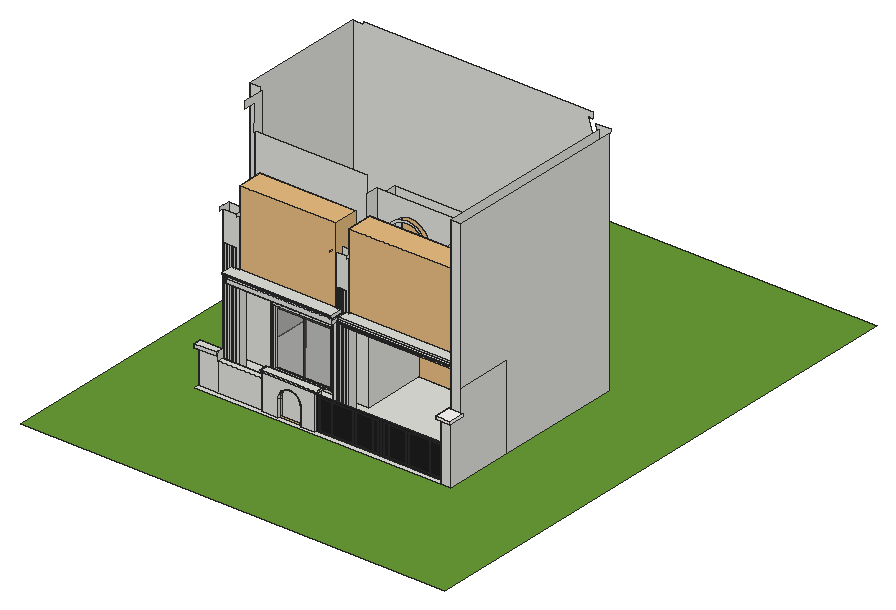
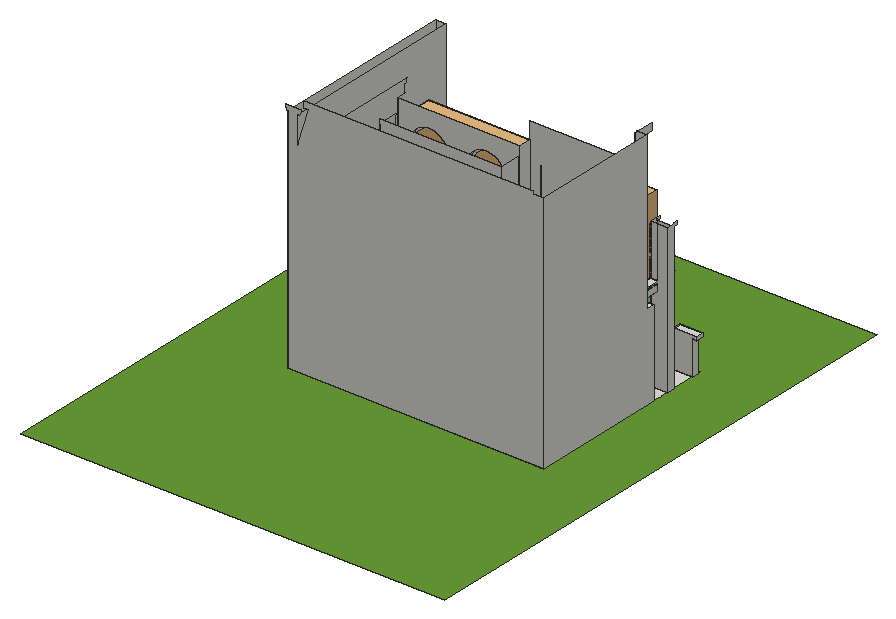
# SketchUp Ruby script. Lengths in millimetres.
U = 1.mm
M = Sketchup.active_model
def pt(a) = Geom::Point3d.new(a.map { |v| v * U })
def face(e, loops, mat)
  f = e.add_face(loops[0].map { |a| pt(a) })
  loops[1..].each { |l| e.add_face(l.map { |a| pt(a) }).erase! }
  f.material = f.back_material = mat if mat
  f
end
# faces: each face lists its corners as indices into pts; further lists are holes
def faces(e, pts, list, mat = nil) = list.each { |f| face(e, (f[0].is_a?(Array) ? f : [f]).map { |l| l.map { |i| pts[i] } }, mat) }
# xy, xz, yz: faces in a plane at the given z, y or x. An outline is a flat list of corners, or four numbers for a rectangle; further outlines are holes
def ring(l) = l.size == 4 ? [[l[0], l[1]], [l[2], l[1]], [l[2], l[3]], [l[0], l[3]]] : l.each_slice(2).to_a
def flat(e, list, mat, &to3) = list.each { |f| face(e, (f[0].is_a?(Array) ? f : [f]).map { |l| ring(l).map { |u, v| to3.(u, v) } }, mat) }
def xy(e, z, list, mat = nil) = flat(e, list, mat) { |x, y| [x, y, z] }
def xz(e, y, list, mat = nil) = flat(e, list, mat) { |x, z| [x, y, z] }
def yz(e, x, list, mat = nil) = flat(e, list, mat) { |y, z| [x, y, z] }
def lines(e, pts, list) = list.each { |a, b| e.add_line(pt(pts[a]), pt(pts[b])) }
# prism: a flat outline (further loops are holes) pulled along v
def prism(e, loops, v, mat = nil)
  f = face(e, loops, mat); d = Geom::Vector3d.new(v.map { |x| x * U })
  f.pushpull(f.normal.samedirection?(d) ? d.length : -d.length)
end
def box(e, o, s, mat = nil) = prism(e, [[o, [o[0] + s[0], o[1], o[2]], [o[0] + s[0], o[1] + s[1], o[2]], [o[0], o[1] + s[1], o[2]]]], [0, 0, s[2]], mat)
def at(x, y, z, deg = 0) = Geom::Transformation.translation(pt([x, y, z])) * Geom::Transformation.rotation(ORIGIN, Z_AXIS, deg.degrees)
def axes(o, x, y, z) = Geom::Transformation.new([*x, 0, *y, 0, *z, 0, *pt(o).to_a, 1])
def part(name) = M.definitions.add(name)
# library, detail: a bought-in or finely detailed component or shape, given as its bounding box
def library(name, o, s) = part(name).tap { |d| box(d.entities, o, s) }
def detail(e, o, s) = box(e.add_group.entities, o, s)
def put(e, d, t, mat = nil) = e.add_instance(d, t).tap { |i| i.material = mat if mat }
def group(e, t, mat = nil) = e.add_group.tap { |g| g.transformation = t; g.material = mat if mat }.entities
root = M.entities
M.materials.add("[0010_Snow]").color = [255, 250, 250]
M.materials.add("[Asphalt New]").color = [67, 60, 62]
M.materials.add("[Color M08]").color = [30, 30, 30]
M.materials.add("[Grass Dark Green]").color = [106, 157, 55]
M.materials.add("[Translucent Glass Gray]").color = [128, 128, 128]
M.materials["[Translucent Glass Gray]"].alpha = 0.5
M.materials.add("[Wood Floor]").color = [155, 105, 61]
M.materials.add("[Wood OSB]").color = [240, 195, 122]
c1 = part("Group\#102")
g1 = group(c1.entities,at(0,0,0))
prism(g1,[[[0,76.2,1828.8],[1790.7,76.2,1828.8],[1790.7,76.2,0],[0,76.2,0]],[[1714.5,76.2,76.2],[1714.5,76.2,1752.6],[76.2,76.2,1752.6],[76.2,76.2,76.2]]],[0,-76.2,0])
c2 = part("Group\#135")
box(c2.entities,[0,0,0],[12.7,25.4,1676.4])
c3 = part("Double driveway gate")
g2 = group(c3.entities,at(1790.7,0,0),"[Color M08]")
put(g2,c1,axes([1790.7,0,0],[-1,0,0],[0,1,0],[0,0,1]))
g3 = group(g2,at(76.2,50.8,76.2))
g4 = group(g3,at(0,-25.4,0))
box(g4,[0,0,0],[139.8,25.4,1676.4])
box(g4,[1291.2,0,0],[347.1,25.4,1676.4])
box(g4,[712.6,0,0],[565.9,25.4,1676.4])
box(g4,[626.3,0,0],[73.6,25.4,1676.4])
box(g4,[152.5,0,0],[461.1,25.4,1676.4])
put(g3,c2,axes([1278.5,0,0],[1,0,0],[0,-1,0],[0,0,1]))
put(g3,c2,axes([613.6,0,0],[1,0,0],[0,-1,0],[0,0,1]))
put(g3,c2,axes([699.9,0,0],[1,0,0],[0,-1,0],[0,0,1]))
put(g3,c2,axes([139.8,0,0],[1,0,0],[0,-1,0],[0,0,1]))
g5 = group(c3.entities,at(1790.7,0,0),"[Color M08]")
put(g5,c1,at(-1790.7,0,0))
g6 = group(g5,at(-76.2,50.8,76.2,-180))
g7 = group(g6,at(0,25.4,0))
box(g7,[0,-25.4,0],[139.8,25.4,1676.4])
box(g7,[1291.2,-25.4,0],[347.1,25.4,1676.4])
box(g7,[712.6,-25.4,0],[565.9,25.4,1676.4])
box(g7,[626.3,-25.4,0],[73.6,25.4,1676.4])
box(g7,[152.5,-25.4,0],[461.1,25.4,1676.4])
put(g6,c2,at(1278.5,0,0))
put(g6,c2,at(613.6,0,0))
put(g6,c2,at(699.9,0,0))
put(g6,c2,at(139.8,0,0))
c4 = library("Glazed entrance door",[0,-35,0],[1000,80.2,2000])
c5 = library("escalier+0",[0,-20,30],[1600,1520,2232])
xy(root,0,[[18830,7763.7,19424.7,7763.7,19424.7,19554.1,4179.9,19554.1,4179.9,11364.2,11672.4,11364.2,11672.4,15798,13910.6,15798,13910.6,15291.6,14018.3,15291.6,14018.3,15102.7,18830,15102.7],[4179.9,7763.7,18830,7763.7,18830,8093.7,11165.5,8093.7,11165.5,7988.9,10315.5,7988.9,10315.5,8071.5,8985.2,8071.5,8985.2,7988.9,8014.2,7988.9,8014.2,8093.7,4179.9,8093.7],[11165.5,8093.7,18830,8932],[[4179.9,8420.8,11165.5,8420.8,11165.5,8932,18830,8932,18830,15102.7,13910.6,15102.7,13910.6,15291.6,11672.4,15291.6,11672.4,11364.2,9781,11364.2,9781,11351.5,9666.6,11351.5,9666.6,11288,5975.6,11288,5975.6,11351.5,5861.2,11351.5,5861.2,11364.2,4179.9,11364.2,4179.9,10323.8,5191.1,10323.8,5191.1,9852.4,4980.7,9852.4,4980.7,10104.8,4850.6,10104.8,4850.6,9852.4,4702.2,9852.4,4702.2,10104.8,4585.1,10104.8,4585.1,9852.4,4415.9,9852.4,4415.9,10085.7,4330.2,10085.7,4330.2,9852.4,4179.9,9852.4],[10715.6,9852.4,10715.6,10323.8,11726.9,10323.8,11726.9,9852.4,11548,9852.4,11548,9993.6,11425.8,9993.6,11425.8,9852.4,11289.9,9852.4,11289.9,10007.9,11185.3,10007.9,11185.3,9852.4,11053.6,9852.4,11053.6,10033.3,10956.8,10033.3,10956.8,9852.4]],[4179.9,9852.4,4330.2,9852.4,4330.2,10085.7,4415.9,10085.7,4415.9,9852.4,4585.1,9852.4,4585.1,10104.8,4702.2,10104.8,4702.2,9852.4,4850.6,9852.4,4850.6,10104.8,4980.7,10104.8,4980.7,9852.4,5191.1,9852.4,5191.1,10323.8,4179.9,10323.8],
  [5975.6,11288,9666.6,11364.2],[5861.2,11351.5,5975.6,11364.2],[9666.6,11351.5,9781,11364.2],[13910.6,15102.7,14018.3,15291.6],[11672.4,15291.6,13910.6,15798]])
xy(root,0,[[[0,0,25274.6,32180.2],[4179.9,7763.7,4179.9,8093.7,8014.2,8093.7,8014.2,7988.9,8985.2,7988.9,8985.2,8071.5,10315.5,8071.5,10315.5,7988.9,11165.5,7988.9,11165.5,8420.8,4179.9,8420.8,4179.9,19554.1,19424.7,19554.1,19424.7,7763.7]]],"[Grass Dark Green]")
xy(root,66,[[9051.2,8071.5,10249.5,8133.4]],"[Wood OSB]")
xy(root,122.4,[[6098,11288,9544.2,11335.6]])
xy(root,199.8,[[6175.4,11335.6,9466.7,11364.2]])
xy(root,359.4,[[15054.6,15102.7,17168.6,15225]])
xy(root,478.1,[[15173.4,15225,17049.8,15291.6]])
xy(root,1708.2,[[5311.7,8093.7,8014.2,8420.8]])
xy(root,2001,[[3987.8,7966.7,5311.7,8093.7],[3987.8,8093.7,4179.9,8420.8]])
xy(root,2102.1,[[7968.2,7949.2,7968.2,8093.7,8014.2,8093.7,8014.2,7988.9,11165.5,7988.9,11165.5,8093.7,11262.4,8093.7,11262.4,7949.2],[7968.2,8093.7,8014.2,8420.8],[11165.5,8093.7,11262.4,8420.8]])
xy(root,2185.3,[[7917.4,7919.1,11392.6,7949.2],[7917.4,7949.2,7968.2,8420.8],[11262.4,7949.2,11392.6,8420.8]])
xy(root,2213,[[7917.4,7919.1,11392.6,8420.8],[3987.8,7966.7,5311.7,8420.8]])
xy(root,3491.1,[[6175.4,11335.6,9466.7,11364.2]])
xy(root,3501.3,[[18683.9,7590.7,18830,8551.1],[18830,7590.7,19424.7,7763.7],[19424.7,7590.7,19532.6,8551.1]])
xy(root,3568.6,[[6098,11288,9544.2,11335.6]])
xy(root,3679.7,[[18683.9,7590.7,19532.6,8551.1]],"[0010_Snow]")
xy(root,3690.9,[[5975.6,11288,9666.6,11351.5]])
xy(root,3756.3,[[15173.4,15225,17049.8,15291.6]])
xy(root,3765.6,[[11672.4,15102.7,11780.1,15291.6],[11780.1,15102.7,13910.6,15798],[11672.4,15291.6,11780.1,15798]])
xy(root,3805.4,[[5861.2,11351.5,9781,11364.2]])
xy(root,3873.3,[[11672.4,15102.7,11780.1,15291.6]])
xy(root,3875.1,[[15054.6,15102.7,17168.6,15225]])
xy(root,4860.9,[[11672.4,9994.1,18830,15102.7]],"[Wood Floor]")
xy(root,4981.6,[[11545.3,9700.5,11545.3,11364.2,11672.4,11364.2,11672.4,9994.1,18830,9994.1,18830,9700.5]])
xy(root,5014.6,[[5191.1,11364.2,10815.6,11889.6]])
xy(root,5014.6,[[5191.1,9487.7,10815.6,11364.2]],"[Wood Floor]")
xy(root,5151.1,[[4815.5,9262.3,4815.5,11364.2,5191.1,11364.2,5191.1,9487.7,10815.6,9487.7,10815.6,11364.2,11160.4,11364.2,11160.4,9262.3],[4179.9,11364.2,4815.5,11889.6],[4815.5,11364.2,5191.1,11889.6],[10815.6,11364.2,11160.4,11889.6]])
xy(root,5371.1,[[11545.3,9262.3,18830,9700.5]])
xy(root,5459.8,[[4802.8,9262.3,4815.5,9852.4],[11160.4,9262.3,11216,9852.4]])
xy(root,5528.1,[[11545.3,9136.9,18830,9262.3]])
xy(root,5565.8,[[11545.3,9136.9,18830,9495.7]])
xy(root,5593.4,[[4747.3,9214.7,11271.6,9262.3],[4747.3,9262.3,4802.8,9852.4],[11216,9262.3,11271.6,9852.4],[4747.3,9852.4,4815.5,11889.6],[11160.4,9852.4,11271.6,11364.2],
  [11160.4,11364.2,11271.6,11889.6]])
xy(root,5638,[[4747.3,9152.8,11271.6,9214.7]])
xy(root,5663.2,[[11545.3,9194,18830,9495.7]])
xy(root,5726.3,[[4747.3,9062.3,11271.6,9152.8]])
xy(root,5732,[[11545.3,9194,18830,9194,18830,12124.7,18102.6,12124.7,18102.6,11848.5,15805,11848.5,15805,12124.7,14682.1,12124.7,14682.1,11848.5,12388.2,11848.5,12388.2,12124.7,11545.3,12124.7],[11545.3,12281.7,18830,12281.7,18830,13477.1,14275.5,13477.1,14275.5,14659.8,11972,14659.8,11972,13477.1,11545.3,13477.1]])
xy(root,5760.6,[[4747.3,9062.3,11271.6,9062.3,11271.6,10323.8,10715.6,10323.8,10715.6,10381,5191.1,10381,5191.1,9852.4,4747.3,9852.4],[4747.3,10323.8,5191.1,10323.8,5191.1,10381,10715.6,10381,10715.6,10323.8,11271.6,10323.8,11271.6,11364.2,9713.9,11364.2,9713.9,11161,9599.1,11161,9599.1,11195.9,9482.2,11195.9,9482.2,11161,9386.9,11161,9386.9,11364.2,6306,11364.2,6306,11161,6210.7,11161,6210.7,11195.9,6093.9,11195.9,6093.9,11161,5979,11161,5979,11364.2,4869.5,11364.2,4869.5,11889.6,4747.3,11889.6],[5979,11161,6093.9,11364.2],[6210.7,11161,6306,11364.2],[9386.9,11161,9482.2,11364.2],
  [9599.1,11161,9713.9,11364.2],[6093.9,11195.9,6210.7,11364.2],[9482.2,11195.9,9599.1,11364.2],[4869.5,11364.2,11271.6,11889.6]])
xy(root,5839.2,[[12495.4,11848.5,14574.9,12281.7]])
xy(root,5844,[[15917.1,11848.5,17990.5,12281.7]])
xz(root,7590.7,[[18683.9,3501.3,19532.6,3679.7]],"[0010_Snow]")
xz(root,7763.7,[[18830,0,19424.7,3501.3]])
xz(root,7919.1,[[7917.4,2185.3,11392.6,2213]])
xz(root,7949.2,[[7968.2,2102.1,11262.4,2185.3]])
xz(root,7966.7,[[3987.8,2001,5311.7,2213]])
xz(root,7988.9,[[8014.2,0,8985.2,0,8985.2,1044.4,9007.8,1216.5,9074.3,1377,9150.6,1476.4,9180,1514.7,9317.7,1620.4,9478.2,1686.9,9650.3,1709.5,9822.5,1686.9,9982.9,1620.4,10120.7,1514.7,10150.1,1476.4,10226.4,1377,10292.8,1216.5,10315.5,1044.4,10315.5,0,11165.5,0,11165.5,2102.1,8014.2,2102.1]])
xz(root,8071.5,[[[8985.2,0,10315.5,0,10315.5,1044.4,10292.8,1216.5,10226.4,1377,10150.1,1476.4,10120.7,1514.7,9982.9,1620.4,9822.5,1686.9,9650.3,1709.5,9478.2,1686.9,9317.7,1620.4,9180,1514.7,9150.6,1476.4,9074.3,1377,9007.8,1216.5,8985.2,1044.4],[9051.2,66,9051.2,1040.1,9072.2,1199.3,9132,1343.7,9202.9,1436.2,9227.1,1467.6,9351,1562.8,9495.4,1622.5,9650.3,1642.9,9805.2,1622.5,9949.6,1562.8,10073.6,1467.6,10097.7,1436.2,10168.7,1343.7,10228.5,1199.3,10249.5,1040.1,10249.5,66]]],"[Wood OSB]")
xz(root,8093.7,[[4179.9,0,5311.7,2001],[5311.7,0,8014.2,1708.2]])
xz(root,8133.4,[[9051.2,66,10249.5,66,10249.5,1040.1,10228.5,1199.3,10168.7,1343.7,10097.7,1436.2,10073.6,1467.6,9949.6,1562.8,9805.2,1622.5,9650.3,1642.9,9495.4,1622.5,9351,1562.8,9227.1,1467.6,9202.9,1436.2,9132,1343.7,9072.2,1199.3,9051.2,1040.1]])
xz(root,8420.8,[[4179.9,0,4179.9,2001,3987.8,2001,3987.8,2213,5311.7,2213,5311.7,1708.2,8014.2,1708.2,8014.2,2102.1,7968.2,2102.1,7968.2,2185.3,7917.4,2185.3,7917.4,2213,11392.6,2213,11392.6,2185.3,11262.4,2185.3,11262.4,2102.1,11165.5,2102.1,11165.5,0]])
xz(root,8551.1,[[18683.9,3501.3,18830,3679.7],[19424.7,3501.3,19532.6,3679.7],[18830,3679.7,19424.7,13753.6]])
xz(root,9062.3,[[4747.3,5726.3,11271.6,5760.6]])
xz(root,9136.9,[[11545.3,5528.1,18830,5565.8]])
xz(root,9152.8,[[4747.3,5638,11271.6,5726.3]])
xz(root,9194,[[11545.3,5663.2,18830,5732]])
xz(root,9214.7,[[4747.3,5593.4,11271.6,5638]])
xz(root,9262.3,[[4815.5,5151.1,11160.4,5459.8],[11545.3,5371.1,18830,5528.1],[4802.8,5459.8,11216,5593.4]])
xz(root,9487.7,[[5191.1,5014.6,10815.6,5151.1]])
xz(root,9495.7,[[11545.3,5565.8,18830,5663.2]])
xz(root,9700.5,[[11545.3,4981.6,18830,5088.6],[11545.3,5088.6,18830,5371.1]])
xz(root,9852.4,[[4179.9,0,4330.2,6858],[4415.9,0,4585.1,6858],[[4702.2,0,4850.6,6858],[4802.8,5459.8,4815.5,5593.4]],[4980.7,0,5191.1,5760.6],[10715.6,0,10715.6,8713.5,11726.9,8713.5,11726.9,0,11548,0,11548,6872.3,11425.8,6872.3,11425.8,0,11289.9,0,11289.9,6861.6,11185.3,6861.6,11185.3,5593.4,11160.4,5593.4,11160.4,5459.8,11185.3,5459.8,11185.3,0,11053.6,0,11053.6,6858,10956.8,6858,10956.8,0],
  [4802.8,5459.8,4815.5,5593.4],[11160.4,5459.8,11185.3,5593.4],[11185.3,5459.8,11216,5593.4],[11185.3,5593.4,11216,6861.6],[4980.7,5760.6,5191.1,5760.6,5191.1,8639.6,4179.9,8639.6,4179.9,6858,4980.7,6858]])
xz(root,9993.6,[[11425.8,0,11548,6872.3]])
xz(root,9994.1,[[11672.4,4860.9,18830,4981.6]])
xz(root,10007.9,[[11185.3,0,11289.9,6861.6]])
xz(root,10033.3,[[10956.8,0,11053.6,6858]])
xz(root,10085.7,[[4330.2,0,4415.9,6858]])
xz(root,10104.8,[[4585.1,0,4702.2,6858],[4850.6,0,4980.7,6858]])
xz(root,10323.8,[[4179.9,0,4179.9,8794.8,4747.3,8794.8,4747.3,5760.6,5191.1,5760.6,5191.1,0],[10715.6,0,11726.9,5760.6],[4747.3,5760.6,5191.1,8794.8],[10715.6,5760.6,11726.9,8794.8]])
xz(root,11161,[[5979,5760.6,6093.9,5760.6,6093.9,9007,9599.1,9007,9599.1,5760.6,9713.9,5760.6,9713.9,9121.9,5979,9121.9],[6210.7,5760.6,6306,5760.6,6306,8794.9,9386.9,8794.9,9386.9,5760.6,9482.2,5760.6,9482.2,8890.1,6210.7,8890.1]])
xz(root,11195.9,[[6093.9,5760.6,6210.7,5760.6,6210.7,8890.1,9482.2,8890.1,9482.2,5760.6,9599.1,5760.6,9599.1,9007,6093.9,9007]])
xz(root,11288,[[[5975.6,0,9666.6,3690.9],[6098,122.4,9544.2,3568.6]]])
xz(root,11335.6,[[[6098,122.4,9544.2,3568.6],[6175.4,199.8,9466.7,3491.1]]])
xz(root,11351.5,[[5861.2,0,5975.6,0,5975.6,3690.9,9666.6,3690.9,9666.6,0,9781,0,9781,3805.4,5861.2,3805.4]])
xz(root,11364.2,[[5861.2,-114.5,9781,0],[4179.9,0,5861.2,0,5861.2,3805.4,9781,3805.4,9781,0,11672.4,0,11672.4,4981.6,11545.3,4981.6,11545.3,12370.5,4869.5,12370.5,4869.5,5760.6,5979,5760.6,5979,9121.9,9713.9,9121.9,9713.9,5760.6,11271.6,5760.6,11271.6,5593.4,11160.4,5593.4,11160.4,5151.1,10815.6,5151.1,10815.6,5014.6,5191.1,5014.6,5191.1,5151.1,4179.9,5151.1],[5979,5645.7,9713.9,5760.6]])
xz(root,11364.2,[[6306,5760.6,6382.4,5760.6,6382.4,8718.5,9310.6,8718.5,9310.6,5760.6,9386.9,5760.6,9386.9,8794.9,6306,8794.9],[7846.5,5760.6,7934.9,8718.5]],"[Asphalt New]")
xz(root,11364.2,[[6175.4,199.8,9466.7,3491.1],[6382.4,5760.6,7846.5,8718.5],[7934.9,5760.6,9310.6,8718.5]],"[Translucent Glass Gray]")
xz(root,11848.5,[[[12388.2,5732,14682.1,5732,14682.1,9152.2,14670.1,9472.3,14570.4,9776.7,14390.8,10042,14163.1,10232.5,14145.1,10247.6,13852.4,10377.7,13535.2,10422.2,13217.9,10377.7,12925.2,10247.6,12907.2,10232.5,12679.5,10042,12499.9,9776.7,12400.2,9472.3,12388.2,9152.2],[12495.4,5839.2,12495.4,9150.1,12506.8,9453.2,12597.2,9729,12759.9,9969.4,12976,10150.3,12982.5,10155.7,13247.7,10273.5,13535.2,10313.9,13822.6,10273.5,14087.8,10155.7,14094.3,10150.3,14310.4,9969.4,14473.2,9729,14563.5,9453.2,14574.9,9150.1,14574.9,5839.2]],[[15805,5732,18102.6,5732,18102.6,9139.4,18092.9,9462,17994.4,9769.3,17990.5,9775.1,17814.8,10037.4,17568,10245.4,17423.3,10310.1,17273.4,10377.1,16953.8,10422.2,16634.2,10377.1,16484.3,10310.1,16339.6,10245.4,16092.8,10037.4,15917.1,9775.1,15913.2,9769.3,15814.7,9462,15805,9139.4],[15917.1,5844,15917.1,9347.6,15968.2,9601.1,16080.3,9834.2,16246.5,10032.4,16456.4,10183.4,16697.2,10277.9,16953.8,10310.1,17210.4,10277.9,17451.2,10183.4,17661.1,10032.4,17827.3,9834.2,17939.4,9601.1,17990.5,9347.6,17990.5,5844]]])
xz(root,11889.6,[[5191.1,5014.6,10815.6,5014.6,10815.6,5151.1,11160.4,5151.1,11160.4,5593.4,11271.6,5593.4,11271.6,5760.6,4747.3,5760.6,4747.3,5593.4,4815.5,5593.4,4815.5,5151.1,5191.1,5151.1],[4179.9,5151.1,4815.5,5151.1,4815.5,5593.4,4747.3,5593.4,4747.3,5760.6,4869.5,5760.6,4869.5,14284.3,4775.8,14284.3,4775.8,14452.6,4179.9,14452.6]])
xz(root,12124.7,[[11545.3,5732,12388.2,5732,12388.2,9152.2,12400.2,9472.3,12499.9,9776.7,12679.5,10042,12907.2,10232.5,12925.2,10247.6,13217.9,10377.7,13535.2,10422.2,13852.4,10377.7,14145.1,10247.6,14163.1,10232.5,14390.8,10042,14570.4,9776.7,14670.1,9472.3,14682.1,9152.2,14682.1,5732,15805,5732,15805,9139.4,15814.7,9462,15913.2,9769.3,15917.1,9775.1,16092.8,10037.4,16339.6,10245.4,16484.3,10310.1,16634.2,10377.1,16953.8,10422.2,17273.4,10377.1,17423.3,10310.1,17568,10245.4,17814.8,10037.4,17990.5,9775.1,17994.4,9769.3,18092.9,9462,18102.6,9139.4,18102.6,5732,18830,5732,18830,11371.3,11545.3,11371.3]])
xz(root,13477.1,[[11545.3,5732,11972,5732,11972,9853.1,14275.5,9853.1,14275.5,5732,18830,5732,18830,10869.6,11545.3,10869.6]])
xz(root,14659.8,[[11972,5732,14275.5,9853.1]])
xz(root,15102.7,[[[14018.3,0,18830,0,18830,4860.9,11672.4,4860.9,11672.4,3873.3,14018.3,3873.3],[15054.6,359.4,17168.6,3875.1]],[13910.6,0,14018.3,0,14018.3,3873.3,11780.1,3873.3,11780.1,3765.6,13910.6,3765.6],[11672.4,3765.6,11780.1,3873.3]])
xz(root,15225,[[[15054.6,359.4,17168.6,3875.1],[15173.4,478.1,17049.8,3756.3]]])
xz(root,15291.6,[[11672.4,-107.7,14018.3,0],[11672.4,3765.6,11780.1,3873.3]])
xz(root,15291.6,[[[15173.4,478.1,17049.8,3756.3],[15223.5,528.2,16999.8,3706.3]],[16111.6,528.2,16145.9,3706.3]],"[Asphalt New]")
xz(root,15291.6,[[15223.5,528.2,16111.6,3706.3],[16145.9,528.2,16999.8,3706.3]],"[Translucent Glass Gray]")
xz(root,15798,[[11672.4,0,13910.6,3765.6]])
xz(root,19554.1,[[4179.9,0,4179.9,14452.6,4815.5,14452.6,4815.5,14595.5,18485.5,14595.5,18485.5,14236.7,18173.1,14236.7,18830,12141.6,18830,13753.6,18742.6,13753.6,18742.6,13895.1,18683.9,13895.1,18683.9,14035.1,19558,14035.1,19558,13895.1,19486.6,13895.1,19486.6,13753.6,19424.7,13753.6,19424.7,0]])
yz(root,3987.8,[[7966.7,2001,8420.8,2213]])
yz(root,4179.9,[[8093.7,0,8420.8,2001],[9852.4,0,9852.4,8639.6,9646,8639.6,9646,8850.3,9852.4,8850.3,9852.4,8794.8,10323.8,8794.8,10323.8,0],[11364.2,0,11364.2,5151.1,11889.6,5151.1,11889.6,14452.6,19554.1,14452.6,19554.1,0]])
yz(root,4330.2,[[9852.4,0,10085.7,6858]])
yz(root,4415.9,[[9852.4,0,10085.7,6858]])
yz(root,4585.1,[[9852.4,0,10104.8,6858]])
yz(root,4702.2,[[9852.4,0,10104.8,6858]])
yz(root,4802.8,[[9262.3,5459.8,9852.4,5593.4]])
yz(root,4815.5,[[9262.3,5151.1,9262.3,5459.8,9852.4,5459.8,9852.4,5593.4,11889.6,5593.4,11889.6,5151.1]])
yz(root,4850.6,[[9852.4,0,10104.8,6858]])
yz(root,4869.5,[[11364.2,5760.6,11364.2,12370.5,11300.2,12370.5,11300.2,12768.3,11364.2,12768.3,11364.2,13883.8,10648.2,13883.8,10648.2,14284.3,11889.6,14284.3,11889.6,5760.6]])
yz(root,4980.7,[[9852.4,0,10104.8,6858]])
yz(root,5191.1,[[9852.4,0,10323.8,5014.6],[9487.7,5014.6,9852.4,5151.1],[9852.4,5014.6,10323.8,5151.1],[10323.8,5014.6,11364.2,5151.1],[11364.2,5014.6,11889.6,5151.1],
  [9852.4,5151.1,10323.8,5760.6],[9852.4,5760.6,10323.8,5760.6,10323.8,8794.8,9646,8794.8,9646,8639.6,9852.4,8639.6],[10323.8,5760.6,10381,8794.8]])
yz(root,5311.7,[[8093.7,1708.2,8420.8,2213],[7966.7,2001,8093.7,2213]])
yz(root,5861.2,[[11351.5,0,11364.2,3805.4]])
yz(root,5975.6,[[11288,0,11351.5,3690.9]])
yz(root,5979,[[11161,5760.6,11364.2,9121.9]])
yz(root,6093.9,[[11161,5760.6,11195.9,9007]])
yz(root,6098,[[11288,122.4,11335.6,3568.6]])
yz(root,6175.4,[[11335.6,199.8,11364.2,3491.1]])
yz(root,6210.7,[[11161,5760.6,11195.9,8890.1]])
yz(root,6306,[[11161,5760.6,11364.2,8794.9]])
yz(root,7917.4,[[7919.1,2185.3,8420.8,2213]])
yz(root,7968.2,[[7949.2,2102.1,8420.8,2185.3]])
yz(root,8014.2,[[7988.9,0,8093.7,1708.2],[7988.9,1708.2,8420.8,2102.1]])
yz(root,8985.2,[[7988.9,0,8071.5,1044.4]])
yz(root,9051.2,[[8071.5,66,8133.4,1040.1]],"[Wood OSB]")
yz(root,9386.9,[[11161,5760.6,11364.2,8794.9]])
yz(root,9466.7,[[11335.6,199.8,11364.2,3491.1]])
yz(root,9482.2,[[11161,5760.6,11195.9,5877.4]])
yz(root,9544.2,[[11288,122.4,11335.6,3568.6]])
yz(root,9599.1,[[11161,5760.6,11195.9,9007]])
yz(root,9666.6,[[11288,0,11351.5,3690.9]])
yz(root,9713.9,[[11161,5760.6,11364.2,9121.9]])
yz(root,9781,[[11351.5,0,11364.2,3805.4]])
yz(root,10249.5,[[8071.5,66,8133.4,1040.1]],"[Wood OSB]")
yz(root,10315.5,[[7988.9,0,8071.5,1044.4]])
yz(root,10715.6,[[9852.4,0,9852.4,8713.5,9646,8713.5,9646,8794.8,10323.8,8794.8,10323.8,0],[10323.8,5760.6,10381,8794.8]])
yz(root,10815.6,[[9487.7,5014.6,11364.2,5151.1],[11364.2,5014.6,11889.6,5151.1]])
yz(root,10956.8,[[9852.4,0,10033.3,6858]])
yz(root,11053.6,[[9852.4,0,10033.3,6858]])
yz(root,11160.4,[[9262.3,5151.1,11364.2,5151.1,11364.2,5593.4,9852.4,5593.4,9852.4,5459.8,9262.3,5459.8],[11364.2,5151.1,11889.6,5593.4]])
yz(root,11165.5,[[7988.9,0,8420.8,2102.1]])
yz(root,11185.3,[[9852.4,0,10007.9,6861.6]])
yz(root,11216,[[9262.3,5459.8,9852.4,5593.4]])
yz(root,11262.4,[[7949.2,2102.1,8420.8,2185.3]])
yz(root,11271.6,[[9214.7,5593.4,11364.2,5593.4,11364.2,5760.6,9062.3,5760.6,9062.3,5726.3,9152.8,5726.3,9152.8,5638,9214.7,5638],[11364.2,5593.4,11889.6,5760.6]])
yz(root,11289.9,[[9852.4,0,10007.9,6861.6]])
yz(root,11392.6,[[7919.1,2185.3,8420.8,2213]])
yz(root,11425.8,[[9852.4,0,9993.6,6872.3]])
yz(root,11545.3,[[9700.5,4981.6,9700.5,5371.1,9262.3,5371.1,9262.3,5528.1,9136.9,5528.1,9136.9,5565.8,9495.7,5565.8,9495.7,5663.2,9194,5663.2,9194,5732,11364.2,5732,11364.2,4981.6],[11364.2,5732,12124.7,11371.3],[12281.7,5732,13477.1,10869.6]])
yz(root,11548,[[9852.4,0,9993.6,6872.3]])
yz(root,11672.4,[[11364.2,0,15798,0,15798,3765.6,15102.7,3765.6,15102.7,4860.9,11364.2,4860.9],[9994.1,4860.9,11364.2,4981.6]])
yz(root,11726.9,[[9852.4,0,10323.8,0,10323.8,8794.8,9852.4,8794.8,9852.4,8828.1,9646,8828.1,9646,8713.5,9852.4,8713.5]])
yz(root,11780.1,[[15102.7,3765.6,15291.6,3873.3]])
yz(root,11972,[[13477.1,5732,14659.8,9853.1]])
yz(root,12388.2,[[11848.5,5732,12124.7,9152.2]])
yz(root,12495.4,[[11848.5,5839.2,12281.7,9150.1]])
yz(root,13910.6,[[15102.7,0,15798,3765.6]])
yz(root,14275.5,[[13477.1,5732,14659.8,9853.1]])
yz(root,14574.9,[[11848.5,5839.2,12281.7,9150.1]])
yz(root,14682.1,[[11848.5,5732,12124.7,9152.2]])
yz(root,15054.6,[[15102.7,359.4,15225,3875.1]])
yz(root,15173.4,[[15225,478.1,15291.6,3756.3]])
yz(root,15805,[[11848.5,5732,12124.7,9139.4]])
yz(root,15917.1,[[11848.5,5844,12281.7,9347.6]])
yz(root,17049.8,[[15225,478.1,15291.6,3756.3]])
yz(root,17168.6,[[15102.7,359.4,15225,3875.1]])
yz(root,17990.5,[[11848.5,5844,12281.7,9347.6]])
yz(root,18102.6,[[11848.5,5732,12124.7,9139.4]])
yz(root,18683.9,[[7590.7,3501.3,8551.1,3679.7]],"[0010_Snow]")
yz(root,18830,[[7763.7,0,7763.7,3501.3,8551.1,3501.3,8551.1,4981.6,9994.1,4981.6,9994.1,4860.9,11300.2,4860.9,11300.2,0],[11300.2,0,15102.7,4860.9],[8551.1,4981.6,8551.1,13753.6,19554.1,13753.6,19554.1,12141.6,11361,12141.6,11361,12064,11403.8,12064,11403.8,11974,11461,11974,11461,11896,11588,11896,11588,11603.9,11575.3,11603.9,11575.3,11540.8,11557.8,11540.8,11557.8,11443.4,11530.8,11443.4,11530.8,11371.3,12124.7,11371.3,12124.7,5732,9194,5732,9194,5663.2,9495.7,5663.2,9495.7,5565.8,9136.9,5565.8,9136.9,5528.1,9262.3,5528.1,9262.3,5371.1,9700.5,5371.1,9700.5,4981.6],[12124.7,5732,12281.7,10572.8],[12281.7,5732,13477.1,10572.8]])
yz(root,19424.7,[[7763.7,0,11889.6,0,11889.6,4981.6,8551.1,4981.6,8551.1,3501.3,7763.7,3501.3],[11889.6,0,19554.1,0,19554.1,13753.6,8551.1,13753.6,8551.1,4981.6,11889.6,4981.6]])
yz(root,19532.6,[[7590.7,3501.3,8551.1,3679.7]],"[0010_Snow]")
p = [[7821.1,11351.5,3411.4],[7821.1,11335.6,199.8],[7916,11335.6,199.8],[7916,11351.5,3411.4],[9051.2,8133.4,1040.1],[9072.2,8133.4,1199.3],
  [9072.2,8071.5,1199.3],[9051.2,8071.5,1040.1],[10228.5,8133.4,1199.3],[10249.5,8133.4,1040.1],[10249.5,8071.5,1040.1],[10228.5,8071.5,1199.3],
  [9007.8,8071.5,1216.5],[9007.8,7988.9,1216.5],[8985.2,7988.9,1044.4],[8985.2,8071.5,1044.4],[10315.5,8071.5,1044.4],[10315.5,7988.9,1044.4],
  [10292.8,7988.9,1216.5],[10292.8,8071.5,1216.5],[9132,8133.4,1343.7],[9132,8071.5,1343.7],[10168.7,8133.4,1343.7],[10168.7,8071.5,1343.7],
  [9074.3,8071.5,1377],[9074.3,7988.9,1377],[10226.4,7988.9,1377],[10226.4,8071.5,1377],[9202.9,8133.4,1436.2],[9202.9,8071.5,1436.2],
  [10097.7,8133.4,1436.2],[10097.7,8071.5,1436.2],[9150.6,8071.5,1476.4],[9150.6,7988.9,1476.4],[10150.1,7988.9,1476.4],[10150.1,8071.5,1476.4],
  [9227.1,8133.4,1467.6],[9227.1,8071.5,1467.6],[10073.6,8133.4,1467.6],[10073.6,8071.5,1467.6],[9351,8133.4,1562.8],[9351,8071.5,1562.8],
  [9949.6,8133.4,1562.8],[9949.6,8071.5,1562.8],[9180,8071.5,1514.7],[9180,7988.9,1514.7],[10120.7,7988.9,1514.7],[10120.7,8071.5,1514.7],
  [9317.7,8071.5,1620.4],[9317.7,7988.9,1620.4],[9982.9,7988.9,1620.4],[9982.9,8071.5,1620.4],[9495.4,8133.4,1622.5],[9495.4,8071.5,1622.5],
  [9805.2,8133.4,1622.5],[9805.2,8071.5,1622.5],[9478.2,8071.5,1686.9],[9478.2,7988.9,1686.9],[9822.5,7988.9,1686.9],[9822.5,8071.5,1686.9],
  [9650.3,8133.4,1642.9],[9650.3,8071.5,1642.9],[9650.3,8071.5,1709.5],[9650.3,7988.9,1709.5],[11545.3,9700.5,5371.1],[11545.3,9852.4,5371.1],
  [5191.1,10381,5760.6],[5191.1,11164.8,5760.6],[5581.6,11351.5,-279.6],[6255.2,11351.5,-279.6],[6255.2,11351.5,280.4],[9387,11351.5,-279.6],
  [10060.6,11351.5,-279.6],[9387,11351.5,280.4],[6255.2,11351.5,3411.4],[9387,11351.5,3411.4],[7968.2,8420.8,2185.3],[7968.2,8442.9,2185.3]]
faces(root,p,[[0,1,2,3]],"[Asphalt New]")
faces(root,p,[[4,5,6,7],[8,9,10,11],[5,20,21,6],[22,8,11,23],[20,28,29,21],[30,22,23,31],[28,36,37,29],[38,30,31,39],
  [36,40,41,37],[42,38,39,43],[40,52,53,41],[54,42,43,55],[52,60,61,53],[60,54,55,61]],"[Wood OSB]")
faces(root,p,[[12,13,14,15],[16,17,18,19],[24,25,13,12],[19,18,26,27],[32,33,25,24],[27,26,34,35],[44,45,33,32],[35,34,46,47],
  [48,49,45,44],[47,46,50,51],[56,57,49,48],[51,50,58,59],[62,63,57,56],[59,58,63,62]])
lines(root,p,[[64,65],[66,67],[68,69],[69,70],[71,72],[73,71],[74,0],[3,75],[75,73],[70,73],[70,74],[76,77]])
put(root,c3,axes([11165.5,8093.7,0],[2.14006,0,0],[0,1,0],[0,0,1.08]))
put(root,c4,axes([11672.4,15196.2,0],[2.23817,0,0],[0,2.232,0],[0,0,1.86]))
put(root,c4,axes([12037.3,13477.1,5732],[2.23817,0,0],[0,2.232,0],[0,0,2.06057]))
put(root,c5,axes([5191.1,9852.4,5730.6],[3.58,0,0],[0,1,0],[0,0,2]))
put(root,c5,axes([11726.9,9852.4,5730.6],[4.4392,0,0],[0,1,0],[0,0,2]))
